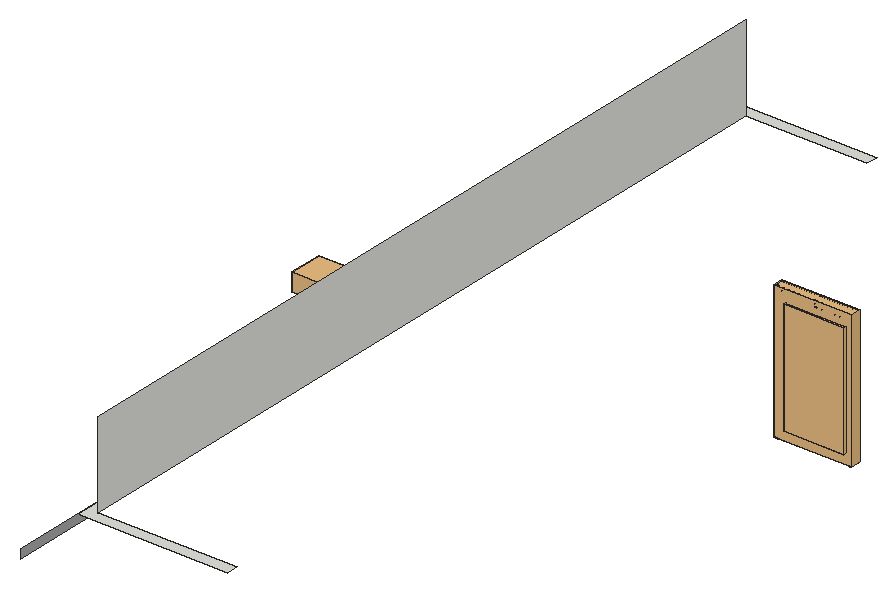
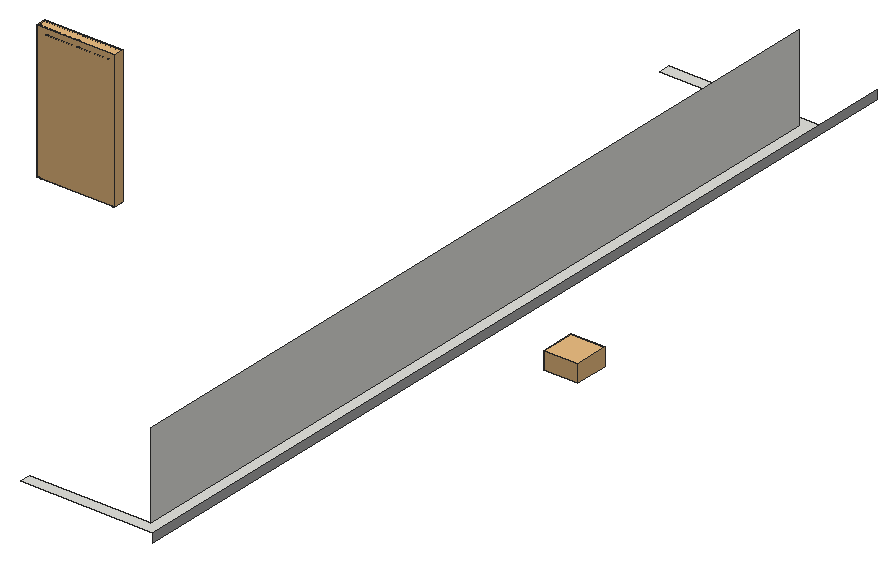
# SketchUp Ruby script. Lengths in inches.
U = 1.inch
M = Sketchup.active_model
def pt(a) = Geom::Point3d.new(a.map { |v| v * U })
def face(e, loops, mat)
  f = e.add_face(loops[0].map { |a| pt(a) })
  loops[1..].each { |l| e.add_face(l.map { |a| pt(a) }).erase! }
  f.material = f.back_material = mat if mat
  f
end
# faces: each face lists its corners as indices into pts; further lists are holes
def faces(e, pts, list, mat = nil) = list.each { |f| face(e, (f[0].is_a?(Array) ? f : [f]).map { |l| l.map { |i| pts[i] } }, mat) }
# xy, xz, yz: faces in a plane at the given z, y or x. An outline is a flat list of corners, or four numbers for a rectangle; further outlines are holes
def ring(l) = l.size == 4 ? [[l[0], l[1]], [l[2], l[1]], [l[2], l[3]], [l[0], l[3]]] : l.each_slice(2).to_a
def flat(e, list, mat, &to3) = list.each { |f| face(e, (f[0].is_a?(Array) ? f : [f]).map { |l| ring(l).map { |u, v| to3.(u, v) } }, mat) }
def xy(e, z, list, mat = nil) = flat(e, list, mat) { |x, y| [x, y, z] }
def xz(e, y, list, mat = nil) = flat(e, list, mat) { |x, z| [x, y, z] }
def yz(e, x, list, mat = nil) = flat(e, list, mat) { |y, z| [x, y, z] }
def lines(e, pts, list) = list.each { |a, b| e.add_line(pt(pts[a]), pt(pts[b])) }
# prism: a flat outline (further loops are holes) pulled along v
def prism(e, loops, v, mat = nil)
  f = face(e, loops, mat); d = Geom::Vector3d.new(v.map { |x| x * U })
  f.pushpull(f.normal.samedirection?(d) ? d.length : -d.length)
end
def box(e, o, s, mat = nil) = prism(e, [[o, [o[0] + s[0], o[1], o[2]], [o[0] + s[0], o[1] + s[1], o[2]], [o[0], o[1] + s[1], o[2]]]], [0, 0, s[2]], mat)
def at(x, y, z, deg = 0) = Geom::Transformation.translation(pt([x, y, z])) * Geom::Transformation.rotation(ORIGIN, Z_AXIS, deg.degrees)
def axes(o, x, y, z) = Geom::Transformation.new([*x, 0, *y, 0, *z, 0, *pt(o).to_a, 1])
def part(name) = M.definitions.add(name)
# library, detail: a bought-in or finely detailed component or shape, given as its bounding box
def library(name, o, s) = part(name).tap { |d| box(d.entities, o, s) }
def detail(e, o, s) = box(e.add_group.entities, o, s)
def put(e, d, t, mat = nil) = e.add_instance(d, t).tap { |i| i.material = mat if mat }
def group(e, t, mat = nil) = e.add_group.tap { |g| g.transformation = t; g.material = mat if mat }.entities
root = M.entities
M.materials.add("Material \#0").color = [86, 53, 35]
M.materials.add("Material \#1").color = [140, 140, 140]
M.materials.add("[0132_LightGray]").color = [169, 169, 169]
c1 = library("Dome Light",[-12,-12,0],[24,24,12])
c2 = part("3DGeom~18_Defintion")
xz(c2.entities,-241.71,[[-976.3,0,23.7,0,23.7,7.58],[-976.3,0,23.7,7.58,-976.3,7.58]],"Material \#0")
xz(c2.entities,241.71,[[-976.3,0,-976.3,7.58,23.7,7.58],[-976.3,0,23.7,7.58,23.7,0]],"Material \#0")
yz(c2.entities,23.7,[[-241.71,0,0,0,-241.71,7.58],[0,0,0,7.58,-241.71,7.58],[0,0,241.71,0,241.71,7.58],[0,0,241.71,7.58,0,7.58]],"Material \#0")
c3 = part("3DGeom~20_Defintion")
xy(c3.entities,0,[[-976.3,-241.71,-976.3,-223.46,23.7,-241.71],[23.7,-241.71,-976.3,-223.46,5.45,-223.46],[23.7,-241.71,5.45,-223.46,5.45,0],[23.7,-241.71,5.45,0,23.7,0],[-976.3,-223.46,-976.3,-211.85,5.45,-223.46],
  [5.45,-223.46,-976.3,-211.85,-6.16,-211.85],[5.45,-223.46,-6.16,-211.85,-6.16,0],[5.45,-223.46,-6.16,0,5.45,0],[-6.16,0,-6.16,211.85,5.45,223.46],[-6.16,0,5.45,223.46,5.45,0],
  [5.45,0,23.7,241.71,23.7,0],[5.45,0,5.45,223.46,23.7,241.71],[-976.3,211.85,-976.3,223.46,5.45,223.46],[-976.3,211.85,5.45,223.46,-6.16,211.85],[-976.3,223.46,-976.3,241.71,23.7,241.71],
  [-976.3,223.46,23.7,241.71,5.45,223.46]],"Material \#0")
c4 = part("3DGeom~22_Defintion")
xz(c4.entities,-210.625,[[-1016.13,2.47,-1016.13,9.96,-16.28,2.47],[-16.28,2.47,-1016.13,9.96,-16.28,9.96],[-1016.13,9.96,-1016.13,51.7,-16.28,51.7],[-1016.13,9.96,-16.28,51.7,-16.28,9.96],[-1016.13,51.7,-1016.13,72.71,-16.28,51.7]],"Material \#0")
xz(c4.entities,210.625,[[-1016.13,2.47,-16.28,2.47,-1016.13,9.96],[-16.28,2.47,-16.28,9.96,-1016.13,9.96],[-1016.13,9.96,-16.28,51.7,-1016.13,51.7],[-1016.13,9.96,-16.28,9.96,-16.28,51.7],[-1016.13,51.7,-16.28,51.7,-1016.13,72.71]],"Material \#0")
yz(c4.entities,-16.28,[[-210.625,2.47,-210.625,9.96,0,9.96],[-210.625,2.47,0,9.96,0,2.47],[0,2.47,0,9.96,210.625,2.47],[210.625,2.47,0,9.96,210.625,9.96],[-210.625,9.96,-210.625,51.7,0,51.7],
  [-210.625,9.96,0,51.7,0,9.96],[0,9.96,0,51.7,210.625,9.96],[210.625,9.96,0,51.7,210.625,51.7],[-210.625,51.7,0,72.71,0,51.7],[0,51.7,0,72.71,210.625,51.7]],"Material \#0")
p = [[-1016.13,-210.625,72.71],[-16.13,-210.77,73.09],[-16.28,-210.625,51.7],[-16.28,-210.625,51.7],[-16.13,-210.77,73.09],[-16.28,0,72.71],
  [-16.13,210.77,73.09],[-16.28,210.625,51.7],[-16.28,210.625,51.7],[-16.13,210.77,73.09],[-1016.13,210.625,72.71]]
faces(c4.entities,p,[[0,1,2],[3,4,5],[5,6,7],[8,9,10]],"Material \#0")
c5 = part("3DGeom~21_Defintion")
xy(c5.entities,73.08,[[-976.3,-241.71,23.7,-241.71,-976.3,-223.46],[23.7,-241.71,5.45,-223.46,-976.3,-223.46],[23.7,-241.71,23.7,0,5.45,-223.46],[5.45,-223.46,23.7,0,5.45,0],[23.7,0,23.7,241.71,5.45,223.46],
  [5.45,0,23.7,0,5.45,223.46],[-976.3,223.46,23.7,241.71,-976.3,241.71],[-976.3,223.46,5.45,223.46,23.7,241.71]],"Material \#0")
c6 = part("3DGeom~19_Defintion")
xy(c6.entities,0,[[-6.28,-215.79,-994.45,-208.55,-13.52,-208.55],[-994.45,-215.79,-994.45,-208.55,-6.28,-215.79],[-6.28,-215.79,-13.52,-208.55,-13.52,0],[-6.28,-215.79,-13.52,0,-6.28,0],[-13.52,0,-13.52,208.55,-6.28,215.79],
  [-13.52,0,-6.28,215.79,-6.28,0],[-994.45,208.55,-6.28,215.79,-13.52,208.55],[-994.45,208.55,-994.45,215.79,-6.28,215.79]],"Material \#0")
p = [[-13.52,-208.55,0],[-994.45,-208.55,0],[-994.45,-207.81,0.07],[-14.25,-207.81,0.07],[-13.52,-208.55,0],[-14.25,-207.81,0.07],
  [-14.25,0,0.07],[-13.52,0,0],[-13.52,208.55,0],[-14.25,207.81,0.07],[-13.52,208.55,0],[-14.25,207.81,0.07],
  [-994.45,207.81,0.07],[-994.45,208.55,0],[-994.45,-207.21,0.27],[-994.45,-207.21,0.27],[-14.86,-207.21,0.27],[-14.86,-207.21,0.27],
  [-14.86,0,0.27],[-14.86,0,0.27],[-14.86,0,0.27],[-14.86,0,0.27],[-14.86,207.21,0.27],[-14.86,207.21,0.27],
  [-994.45,207.21,0.27],[-994.45,207.21,0.27],[-14.86,-207.21,0.27],[-994.45,-207.21,0.27],[-994.45,-206.74,0.6],[-15.33,-206.74,0.6],
  [-14.86,-207.21,0.27],[-15.33,-206.74,0.6],[-15.33,0,0.6],[-14.86,0,0.27],[-14.86,207.21,0.27],[-15.33,206.74,0.6],
  [-14.86,207.21,0.27],[-15.33,206.74,0.6],[-994.45,206.74,0.6],[-994.45,207.21,0.27],[-994.45,-206.4,1.07],[-15.66,-206.4,1.07],
  [-15.66,-206.4,1.07],[-15.66,0,1.07],[-15.66,206.4,1.07],[-15.66,206.4,1.07],[-994.45,206.4,1.07],[-994.45,-206.2,1.68],
  [-15.86,-206.2,1.68],[-15.86,-206.2,1.68],[-15.86,0,1.68],[-15.86,206.2,1.68],[-15.86,206.2,1.68],[-994.45,206.2,1.68],
  [-994.45,-206.13,2.41],[-15.93,-206.13,2.41],[-15.93,-206.13,2.41],[-15.93,0,2.41],[-15.93,206.13,2.41],[-15.93,206.13,2.41],
  [-994.45,206.13,2.41],[-994.45,-206.13,71.16],[-994.45,-206.22,71.59],[-15.79,-206.28,71.53],[-15.79,-206.28,71.53],[-15.84,0,71.59],
  [-15.93,0,71.16],[-15.79,206.28,71.53],[-15.79,206.28,71.53],[-994.45,206.22,71.59],[-994.45,206.13,71.16],[-15.79,-206.28,71.53],
  [-994.45,-206.48,71.84],[-994.45,-206.9,71.93],[-15.16,-206.9,71.93],[-15.79,-206.28,71.53],[-15.79,-206.28,71.53],[-15.16,-206.9,71.93],
  [-15.16,0,71.93],[-994.45,-206.48,71.84],[-15.59,0,71.84],[-15.79,-206.28,71.53],[-15.59,0,71.84],[-15.79,206.28,71.53],
  [-15.16,206.9,71.93],[-15.59,0,71.84],[-15.79,206.28,71.53],[-994.45,206.48,71.84],[-15.79,206.28,71.53],[-15.16,206.9,71.93],
  [-994.45,206.9,71.93],[-994.45,206.48,71.84],[-15.79,206.28,71.53],[-994.45,-227.27,72.01],[5.41,-227.47,72.33],[4.78,-226.84,71.93],
  [4.78,-226.84,71.93],[5.41,-227.47,72.33],[5.21,0,72.01],[-994.45,-226.84,71.93],[-994.45,-227.27,72.01],[5.21,0,72.01],
  [4.78,0,71.93],[4.78,226.84,71.93],[5.21,0,72.01],[5.21,0,72.01],[5.41,227.47,72.33],[4.78,226.84,71.93],
  [5.41,227.47,72.33],[-994.45,227.27,72.01],[-994.45,227.27,72.01],[-994.45,226.84,71.93],[-994.45,-227.27,72.01],[-994.45,-227.53,72.27],
  [5.41,-227.47,72.33],[5.41,-227.47,72.33],[5.47,0,72.27],[5.21,0,72.01],[5.41,227.47,72.33],[5.41,227.47,72.33],
  [-994.45,227.53,72.27],[-994.45,227.27,72.01],[-994.45,-227.61,72.7],[-994.45,-227.61,74.4375],[-994.45,-227.61,74.4375],[5.55,-227.61,74.4375],
  [5.55,-227.61,74.4375],[5.55,0,74.4375],[5.55,0,72.7],[5.55,227.61,74.4375],[5.55,227.61,74.4375],[-994.45,227.61,74.4375],
  [-994.45,227.61,74.4375],[-994.45,227.61,72.7]]
faces(c6.entities,p,[[0,1,2],[2,3,0],[4,5,6],[6,7,4],[8,7,6],[6,9,8],[10,11,12],[12,13,10],
  [3,2,14],[15,16,3],[5,17,18],[19,6,5],[9,6,20],[21,22,9],[11,23,24],[25,12,11],
  [26,27,28],[28,29,26],[30,31,32],[32,33,30],[34,33,32],[32,35,34],[36,37,38],[38,39,36],
  [29,28,40],[40,41,29],[31,42,43],[43,32,31],[35,32,43],[43,44,35],[37,45,46],[46,38,37],
  [41,40,47],[47,48,41],[42,49,50],[50,43,42],[44,43,50],[50,51,44],[45,52,53],[53,46,45],
  [48,47,54],[54,55,48],[49,56,57],[57,50,49],[51,50,57],[57,58,51],[52,59,60],[60,53,52],
  [61,62,63],[64,65,66],[66,65,67],[68,69,70],[71,72,73],[73,74,75],[76,77,78],[62,79,63],
  [78,80,76],[81,82,65],[83,80,78],[78,84,83],[65,85,86],[68,87,69],[88,89,90],[90,91,92],
  [93,94,95],[96,97,98],[95,99,100],[101,102,96],[103,102,104],[105,106,103],[107,108,109],[110,111,107],
  [112,113,114],[115,116,117],[117,116,118],[119,120,121],[114,122,123],[124,125,114],[113,122,114],[115,126,127],
  [127,128,115],[115,128,116],[118,128,127],[127,129,118],[116,128,118],[119,130,131],[132,133,119],[119,133,120]],"Material \#0")
c7 = part("3DGeom~15_Defintion")
xy(c7.entities,0,[[-961.58,-251.9,-958.5,-248.8125,-961.58,-237.8],[-961.58,-251.9,28.8,-248.8125,-958.5,-248.8125],[-961.58,-251.9,36.25,-251.9,28.8,-248.8125],[36.25,-251.9,19.98,-239.99,28.8,-248.8125],[36.25,-251.9,22.16,-237.8,19.98,-239.99],
  [-958.5,-248.8125,-958.5,-237.8,-961.58,-237.8],[19.98,-239.99,22.16,-237.8,3.36,-223.37],[-958.5,-237.8,-958.5,-223.37,-961.58,-220.28],[-961.58,-237.8,-958.5,-237.8,-961.58,-220.28],[22.16,-237.8,4.64,-220.28,3.36,-223.37],
  [-958.5,-223.37,4.64,-220.28,-961.58,-220.28],[-958.5,-223.37,3.36,-223.37,4.64,-220.28],[5.29,-219.63,8.375,-218.35,5.29,0],[8.375,-218.35,8.375,0,5.29,0],[5.29,0,8.375,0,5.29,219.63],
  [8.375,0,8.375,218.35,5.29,219.63],[8.375,218.35,22.8125,237.15,5.29,219.63],[-961.58,220.28,-958.5,223.37,-961.58,237.8],[-961.58,220.28,3.36,223.37,-958.5,223.37],[-961.58,220.28,4.64,220.28,3.36,223.37],
  [4.64,220.28,19.98,239.99,3.36,223.37],[4.64,220.28,22.16,237.8,19.98,239.99],[-958.5,223.37,-958.5,237.8,-961.58,237.8],[-958.5,237.8,-958.5,248.8125,-961.58,251.9],[-961.58,237.8,-958.5,237.8,-961.58,251.9],
  [22.16,237.8,28.8,248.8125,19.98,239.99],[22.16,237.8,36.25,251.9,28.8,248.8125],[-958.5,248.8125,36.25,251.9,-961.58,251.9],[-958.5,248.8125,28.8,248.8125,36.25,251.9]],"Material \#0")
xy(c7.entities,7.48,[[-962.79,-238.36,23.37,-238.36,-962.79,-219.67],[23.37,-238.36,4.67,-219.67,-962.79,-219.67],[23.37,-238.36,23.37,0,4.67,-219.67],[4.67,-219.67,23.37,0,4.67,0],[23.37,0,23.37,238.36,4.67,219.67],
  [4.67,0,23.37,0,4.67,219.67],[-962.79,219.67,23.37,238.36,-962.79,238.36],[-962.79,219.67,4.67,219.67,23.37,238.36]],"Material \#0")
xy(c7.entities,63.5625,[[-962.79,-238.36,-962.79,-219.67,4.67,-219.67],[-962.79,-238.36,4.67,-219.67,23.37,-238.36],[23.37,-238.36,4.67,-219.67,23.37,0],[4.67,-219.67,4.67,0,23.37,0],[23.37,0,4.67,219.67,23.37,238.36],
  [4.67,0,4.67,219.67,23.37,0],[-962.79,219.67,-962.79,238.36,4.67,219.67],[4.67,219.67,-962.79,238.36,23.37,238.36]],"Material \#0")
xy(c7.entities,69.64,[[-962.79,-219.62,4.63,-219.62,-962.79,-200.32],[4.63,-219.62,-14.68,-200.32,-962.79,-200.32],[4.63,-219.62,4.63,0,-14.68,-200.32],[-14.68,-200.32,4.63,0,-14.68,0],[-14.68,0,4.63,0,-14.68,200.32],
  [4.63,0,4.63,219.62,-14.68,200.32],[-962.79,200.32,-14.68,200.32,4.63,219.62],[-962.79,200.32,4.63,219.62,-962.79,219.62]],"Material \#0")
xy(c7.entities,71.04,[[-961.58,-251.9,-958.5,-248.8125,28.8,-248.8125],[-961.58,-251.9,-961.58,-237.8,-958.5,-248.8125],[-961.58,-251.9,28.8,-248.8125,36.25,-251.9],[36.25,-251.9,19.98,-239.99,22.16,-237.8],[36.25,-251.9,28.8,-248.8125,19.98,-239.99],
  [-958.5,-248.8125,-961.58,-237.8,-958.5,-237.8],[19.98,-239.99,3.36,-223.37,22.16,-237.8],[-958.5,-237.8,-961.58,-220.28,-958.5,-223.37],[-961.58,-237.8,-961.58,-220.28,-958.5,-237.8],[22.16,-237.8,3.36,-223.37,4.64,-220.28],
  [-958.5,-223.37,-961.58,-220.28,4.64,-220.28],[-958.5,-223.37,4.64,-220.28,3.36,-223.37],[5.29,-219.63,5.29,0,8.375,-218.35],[8.375,-218.35,5.29,0,8.375,0],[5.29,0,5.29,219.63,8.375,0],
  [8.375,0,5.29,219.63,8.375,218.35],[8.375,218.35,5.29,219.63,22.8125,237.15],[-961.58,220.28,-958.5,223.37,3.36,223.37],[-961.58,220.28,-961.58,237.8,-958.5,223.37],[-961.58,220.28,3.36,223.37,4.64,220.28],
  [4.64,220.28,3.36,223.37,19.98,239.99],[4.64,220.28,19.98,239.99,22.16,237.8],[-958.5,223.37,-961.58,237.8,-958.5,237.8],[-958.5,237.8,-961.58,251.9,-958.5,248.8125],[-961.58,237.8,-961.58,251.9,-958.5,237.8],
  [22.16,237.8,19.98,239.99,28.8,248.8125],[22.16,237.8,28.8,248.8125,36.25,251.9],[-958.5,248.8125,-961.58,251.9,36.25,251.9],[-958.5,248.8125,36.25,251.9,28.8,248.8125]],"Material \#0")
xz(c7.entities,-238.36,[[-962.79,63.5625,23.37,63.5625,23.37,72.07],[-962.79,63.5625,23.37,72.07,-962.79,72.07]],"Material \#0")
xz(c7.entities,-219.67,[[-962.79,7.48,4.67,7.48,-962.79,63.5625],[4.67,7.48,4.67,63.5625,-962.79,63.5625]],"Material \#0")
xz(c7.entities,219.67,[[-962.79,7.48,-962.79,63.5625,4.67,7.48],[4.67,7.48,-962.79,63.5625,4.67,63.5625]],"Material \#0")
xz(c7.entities,238.36,[[-962.79,63.5625,-962.79,72.07,23.37,72.07],[-962.79,63.5625,23.37,72.07,23.37,63.5625]],"Material \#0")
yz(c7.entities,4.67,[[-219.67,7.48,0,7.48,-219.67,63.5625],[0,7.48,0,63.5625,-219.67,63.5625],[0,7.48,219.67,63.5625,0,63.5625],[0,7.48,219.67,7.48,219.67,63.5625]],"Material \#0")
yz(c7.entities,23.37,[[-238.36,63.5625,0,63.5625,-238.36,72.07],[0,63.5625,0,72.07,-238.36,72.07],[0,63.5625,238.36,63.5625,238.36,72.07],[0,63.5625,238.36,72.07,0,72.07]],"Material \#0")
p = [[36.9,-251.24,0],[37.21,0,-0.16],[34.125,0,-0.14],[36.9,251.24,0],[33.83,243.81,0.02],[33.83,-243.8,0.02],
  [22.8125,-237.15,0],[24.99,-234.97,-0.01],[5.375,-220.37,0],[23.37,-238.36,7.48],[4.67,-219.67,7.48],[4.67,-219.67,7.48],
  [23.37,-238.36,7.48],[23.37,-238.36,0],[4.67,-219.67,7.48],[23.37,-238.36,0],[5.375,-220.37,0],[5.375,-220.37,0],
  [23.37,-238.36,0],[5.29,-219.63,0],[8.375,-218.35,0],[-15.36,-199.64,1.62],[4.67,-219.67,7.48],[5.375,-220.37,0],
  [-13.8,-201.19,0.06],[5.375,-220.37,0],[5.375,-220.37,0],[-14.84,-200.15,0.58],[5.375,-220.37,0],[-13.8,-201.19,0.06],
  [-6.08,-208.92,0],[5.375,-220.37,0],[-13.8,-201.19,0.06],[-6.08,-208.92,0],[-13.8,-201.19,0.06],[5.375,-220.37,0],
  [-6.08,-208.92,0],[-13.8,-201.19,0.06],[-13.09,-201.91,0],[-6.08,-208.92,0],[-13.09,-201.91,0],[-13.8,-201.19,0.06],
  [-15.36,199.64,1.62],[4.67,219.67,7.48],[5.375,220.37,0],[-13.8,201.19,0.06],[5.375,220.37,0],[5.375,220.37,0],
  [4.67,219.67,7.48],[-14.84,200.15,0.58],[5.375,220.37,0],[-13.8,201.19,0.06],[-6.08,208.92,0],[-13.09,201.91,0],
  [-13.8,201.19,0.06],[-6.08,208.92,0],[-13.8,201.19,0.06],[5.375,220.37,0],[-6.08,208.92,0],[5.375,220.37,0],
  [-13.8,201.19,0.06],[-6.08,208.92,0],[-13.8,201.19,0.06],[-13.09,201.91,0],[8.375,218.35,0],[24.99,234.97,-0.01],
  [22.8125,237.15,0],[23.37,238.36,7.48],[23.37,238.36,0],[23.37,238.36,0],[5.375,220.37,0],[5.375,220.37,0],
  [23.37,238.36,7.48],[4.67,219.67,7.48],[5.375,220.37,0],[23.37,238.36,0],[23.37,238.36,7.48],[-13.8,-201.19,0.06],
  [-14.84,-200.15,0.58],[-14.38,-200.61,0.26],[-13.8,-201.19,0.06],[-13.8,-201.19,0.06],[-14.38,-200.61,0.26],[-13.8,201.19,0.06],
  [-14.84,200.15,0.58],[-13.8,201.19,0.06],[-14.38,200.61,0.26],[-14.38,200.61,0.26],[-13.8,201.19,0.06],[4.63,-219.62,69.64],
  [4.63,-219.62,69.64],[-15.42,-199.57,9.43],[-15.36,-199.64,1.62],[-15.16,-199.83,1.04],[-15.16,-199.83,1.04],[-15.16,199.83,1.04],
  [-15.36,199.64,1.62],[-15.16,199.83,1.04],[-15.42,199.57,9.43],[4.63,219.62,69.64],[4.67,219.67,7.48],[4.63,219.62,69.64],
  [4.63,-219.62,69.64],[4.67,-219.67,63.5625],[4.67,-219.67,63.5625],[4.67,-219.67,7.48],[-15.28,-199.71,69.25],[4.63,-219.62,69.64],
  [-15.42,-199.57,9.43],[-15.28,-199.71,69.25],[-15.42,-199.57,2.34],[-15.42,-199.57,2.34],[-15.42,199.57,2.34],[-15.42,199.57,9.43],
  [-15.28,199.71,69.25],[-15.28,199.71,69.25],[4.63,219.62,69.64],[4.63,219.62,69.64],[4.67,219.67,63.5625],[4.67,219.67,63.5625],
  [-15.42,199.57,2.34],[4.67,-219.67,63.5625],[4.63,-219.62,69.64],[4.67,219.67,7.48],[4.67,219.67,63.5625],[4.63,219.62,69.64],
  [4.63,-219.62,69.64],[-15.28,-199.71,69.25],[-15.28,-199.71,69.25],[-15.42,-199.57,48.99],[-15.42,-199.57,48.99],[-15.28,-199.71,69.25],
  [-15.42,199.57,48.99],[-15.28,199.71,69.25],[-15.28,199.71,69.25],[-15.42,199.57,48.99],[4.63,219.62,69.64],[4.63,-219.62,69.64],
  [23.37,-238.36,72.07],[4.67,-219.67,63.5625],[4.67,-219.67,63.5625],[23.37,-238.36,63.5625],[23.37,-238.36,72.07],[4.67,-219.67,63.5625],
  [5.24,-220.23,70.03],[23.37,-238.36,72.07],[23.37,-238.36,63.5625],[4.67,-219.67,63.5625],[4.67,-219.67,63.5625],[4.63,-219.62,69.64],
  [4.63,219.62,69.64],[23.37,238.36,72.07],[4.67,219.67,63.5625],[4.67,219.67,63.5625],[5.24,220.23,70.03],[4.63,219.62,69.64],
  [23.37,238.36,63.5625],[4.67,219.67,63.5625],[4.67,219.67,63.5625],[23.37,238.36,63.5625],[23.37,238.36,72.07],[4.67,219.67,63.5625],
  [23.37,238.36,72.07],[4.63,-219.62,69.64],[-14.68,-200.32,69.64],[-15.28,-199.71,69.25],[-15.28,-199.71,69.25],[-14.68,-200.32,69.64],
  [4.63,-219.62,69.64],[-15.28,199.71,69.25],[-14.68,200.32,69.64],[4.63,219.62,69.64],[4.63,219.62,69.64],[-14.68,200.32,69.64],
  [4.63,-219.62,69.64],[5.24,-220.23,70.03],[23.37,-238.36,72.07],[4.63,219.62,69.64],[5.24,220.23,70.03],[5.375,-220.37,72.07],
  [5.375,-220.37,72.07],[23.37,-238.36,72.07],[5.375,220.37,72.07],[23.37,238.36,72.07],[5.375,220.37,72.07],[33.83,-243.8,71.03],
  [36.9,-251.24,71.04],[22.8125,-237.15,71.04],[34.125,0,71.19],[37.21,0,71.2],[24.99,-234.97,71.05],[5.29,-219.63,71.04],
  [8.375,-218.35,71.04],[33.83,243.81,71.03],[36.9,251.24,71.04],[22.8125,237.15,71.04],[24.99,234.97,71.05],[8.375,218.35,71.04]]
faces(c7.entities,p,[[0,1,2],[1,3,4],[4,2,1],[2,5,0],[6,0,5],[5,7,6],[8,9,10],[11,12,13],
  [14,15,16],[17,18,9],[19,6,7],[7,20,19],[21,22,23],[24,21,25],[26,10,27],[28,27,29],
  [30,31,32],[33,34,35],[36,37,38],[39,40,41],[42,43,44],[45,42,46],[47,48,49],[50,49,51],
  [52,53,54],[55,56,57],[58,59,60],[61,62,63],[64,65,66],[43,67,68],[43,69,70],[71,72,73],
  [74,75,76],[3,66,65],[65,4,3],[77,78,21],[27,79,80],[81,82,78],[83,84,42],[85,86,84],
  [49,87,88],[10,89,27],[90,91,27],[92,93,27],[91,92,27],[78,94,21],[84,95,42],[96,97,49],
  [98,96,49],[99,98,49],[100,101,49],[21,102,103],[21,104,105],[21,106,107],[21,108,109],[91,110,92],
  [21,111,108],[42,112,113],[42,113,114],[42,115,116],[42,117,118],[42,119,43],[98,120,96],[10,121,122],
  [123,124,125],[126,127,91],[128,129,91],[108,130,131],[113,132,133],[134,135,98],[136,134,98],[137,138,139],
  [140,141,142],[143,142,144],[145,146,147],[148,144,149],[150,151,152],[153,154,155],[151,156,157],[158,159,160],
  [161,162,154],[163,164,165],[166,167,168],[169,170,171],[172,173,134],[174,175,176],[177,178,151],[142,179,144],
  [175,180,181],[178,182,151],[183,184,154],[185,186,187],[186,185,188],[188,189,186],[187,190,185],[190,187,191],
  [191,192,190],[189,188,193],[193,194,189],[195,196,197],[196,195,194],[194,193,196]],"Material \#0")
c8 = library("3DGeom~16_Defintion",[-962.62,-252.34,-11.22],[1000,504.68,93.46])
c9 = part("3DGeom~17_Defintion")
yz(c9.entities,-1908.8,[[-436.03,-21.87,-436.73,-21.5,-435.91,-21.83],[436.03,-21.87,435.91,-21.83,436.73,-21.5],[-435.91,-21.83,-436.73,-21.5,-436.15,-21.125],[-435.91,-21.83,-436.15,-21.125,-435.87,-21.72],[435.91,-21.83,435.87,-21.72,436.15,-21.125],
  [435.91,-21.83,436.15,-21.125,436.73,-21.5],[-436.73,-21.5,-484.73,-21.37,-436.15,-1.11],[-471.46,-21.5,-484.73,-21.37,-436.73,-21.5],[-477.2,-21.5,-484.73,-21.37,-471.46,-21.5],[-481.82,-21.5,-484.73,-21.37,-477.2,-21.5],
  [-436.73,-21.5,-436.15,-1.11,-436.15,-21.125],[436.73,-21.5,436.15,-21.125,471.46,-21.5],[471.46,-21.5,436.15,-21.125,477.2,-21.5],[477.2,-21.5,436.15,-21.125,499.98,-0.85],[477.2,-21.5,499.98,-0.85,481.82,-21.5],
  [481.82,-21.5,487.35,-21,484.73,-21.37],[481.82,-21.5,491.8,-19.52,487.35,-21],[481.82,-21.5,497.64,-13.67,491.8,-19.52],[481.82,-21.5,499.98,-0.85,497.64,-13.67],[-484.73,-21.37,-498.5,-11.58,-499.84,-0.37],
  [-484.73,-21.37,-499.84,-0.37,-499.4,-0.5],[-484.73,-21.37,-499.4,-0.5,-436.15,-1.11],[-484.73,-21.37,-493.63,-18.42,-498.5,-11.58],[-484.73,-21.37,-489.71,-20.375,-493.63,-18.42],[-484.73,-21.37,-487.35,-21,-489.71,-20.375],
  [436.15,-21.125,436.15,-1.11,436.73,-0.74],[436.15,-21.125,436.73,-0.74,499.98,-0.85],[487.35,-21,491.8,-19.52,489.71,-20.375],[-489.71,-20.375,-491.8,-19.52,-493.63,-18.42],[491.8,-19.52,495.21,-17.08,493.63,-18.42],
  [491.8,-19.52,497.64,-13.67,495.21,-17.08],[-493.63,-18.42,-496.54,-15.5,-498.5,-11.58],[-493.63,-18.42,-495.21,-17.08,-496.54,-15.5],[495.21,-17.08,497.64,-13.67,496.54,-15.5],[-496.54,-15.5,-497.64,-13.67,-498.5,-11.58],
  [497.64,-13.67,499.125,-9.22,498.5,-11.58],[497.64,-13.67,499.625,-3.69,499.125,-9.22],[497.64,-13.67,499.98,-0.85,499.625,-3.69],[-498.5,-11.58,-499.625,-3.69,-499.84,-0.37],[-498.5,-11.58,-499.5,-6.6,-499.625,-3.69],
  [-498.5,-11.58,-499.125,-9.22,-499.5,-6.6],[499.125,-9.22,499.625,-3.69,499.5,-6.6],[-499.625,-3.69,-499.98,-0.85,-500,-0.52],[-499.625,-3.69,-500,-0.52,-499.84,-0.37],[-436.15,-1.11,-499.4,-0.5,-471.46,-0.74],
  [-436.15,-1.11,-471.46,-0.74,-436.73,-0.74],[-436.15,-1.11,-436.73,-0.74,-435.91,-0.41],[-436.15,-1.11,-435.91,-0.41,-435.87,-0.52],[436.15,-1.11,435.87,-0.52,435.91,-0.41],[436.15,-1.11,435.91,-0.41,436.73,-0.74],
  [499.98,-0.85,436.73,-0.74,471.46,-0.74],[499.98,-0.85,471.46,-0.74,499.4,-0.5],[499.98,-0.85,499.4,-0.5,499.96,-0.41],[499.98,-0.85,499.96,-0.41,500,-0.52],[-436.73,-0.74,-436.03,-0.37,-435.91,-0.41],
  [436.73,-0.74,435.91,-0.41,436.03,-0.37],[-500,-0.52,-499.96,-0.41,-499.84,-0.37],[499.4,-0.5,499.84,-0.37,499.96,-0.41],[-499.84,141.21,-499.96,141.25,-499.4,141.35],[-436.03,141.21,-436.73,141.59,-435.91,141.25],
  [436.03,141.21,435.91,141.25,436.73,141.59],[499.84,141.21,484.73,162.21,498.5,152.42],[499.84,141.21,499.4,141.35,484.73,162.21],[499.84,141.21,498.5,152.42,499.625,144.53],[499.84,141.21,499.625,144.53,500,141.37],
  [499.84,141.21,500,141.37,499.96,141.25],[-499.96,141.25,-500,141.37,-499.98,141.69],[-499.96,141.25,-499.98,141.69,-499.4,141.35],[-435.91,141.25,-436.73,141.59,-436.15,141.96],[-435.91,141.25,-436.15,141.96,-435.87,141.37],
  [435.91,141.25,435.87,141.37,436.15,141.96],[435.91,141.25,436.15,141.96,436.73,141.59],[-499.4,141.35,-499.98,141.69,-471.46,141.59],[499.4,141.35,436.15,141.96,484.73,162.21],[499.4,141.35,471.46,141.59,436.15,141.96],
  [500,141.37,499.625,144.53,499.98,141.69],[-436.73,141.59,-499.98,141.69,-436.15,161.97],[-471.46,141.59,-499.98,141.69,-436.73,141.59],[-436.73,141.59,-436.15,161.97,-436.15,141.96],[436.73,141.59,436.15,141.96,471.46,141.59],
  [-499.98,141.69,-477.2,162.34,-436.15,161.97],[-499.98,141.69,-481.82,162.34,-477.2,162.34],[-499.98,141.69,-497.64,154.51,-481.82,162.34],[-499.98,141.69,-499.625,144.53,-497.64,154.51],[436.15,141.96,436.15,161.97,436.73,162.34],
  [436.15,141.96,436.73,162.34,484.73,162.21],[-499.625,144.53,-499.125,150.07,-497.64,154.51],[-499.625,144.53,-499.5,147.44,-499.125,150.07],[499.625,144.53,498.5,152.42,499.5,147.44],[499.5,147.44,498.5,152.42,499.125,150.07],
  [-499.125,150.07,-498.5,152.42,-497.64,154.51],[498.5,152.42,484.73,162.21,493.63,159.26],[498.5,152.42,493.63,159.26,496.54,156.34],[498.5,152.42,496.54,156.34,497.64,154.51],[-497.64,154.51,-491.8,160.36,-481.82,162.34],
  [-497.64,154.51,-495.21,157.92,-491.8,160.36],[-497.64,154.51,-496.54,156.34,-495.21,157.92],[496.54,156.34,493.63,159.26,495.21,157.92],[-495.21,157.92,-493.63,159.26,-491.8,160.36],[493.63,159.26,484.73,162.21,489.71,161.22],
  [493.63,159.26,489.71,161.22,491.8,160.36],[-491.8,160.36,-487.35,161.84,-481.82,162.34],[-491.8,160.36,-489.71,161.22,-487.35,161.84],[489.71,161.22,484.73,162.21,487.35,161.84],[-487.35,161.84,-484.73,162.21,-481.82,162.34],
  [-436.15,161.97,-477.2,162.34,-471.46,162.34],[-436.15,161.97,-471.46,162.34,-436.73,162.34],[-436.15,161.97,-436.73,162.34,-435.91,162.68],[-436.15,161.97,-435.91,162.68,-435.87,162.56],[436.15,161.97,435.87,162.56,435.91,162.68],
  [436.15,161.97,435.91,162.68,436.73,162.34],[484.73,162.21,436.73,162.34,471.46,162.34],[484.73,162.21,471.46,162.34,477.2,162.34],[484.73,162.21,477.2,162.34,481.82,162.34],[-436.73,162.34,-436.03,162.72,-435.91,162.68],
  [436.73,162.34,435.91,162.68,436.03,162.72]],"Material \#0")
c10 = library("3DGeom~6_Defintion",[-5.59,-471.8,-48.03],[468.87,1000,73.72])
xy(root,0,[[1338.625,223.9375,1338.625,807.5,1431.3125,807.5,1431.3125,799.5,1346.625,799.5,1346.625,231.9375,1443.61,231.9375,1443.61,223.9375]])
yz(root,1338.625,[[173.9375,-6,807.5,0]],"[0132_LightGray]")
yz(root,1346.625,[[231.9375,0,799.5,60]])
put(root,c1,at(1280.26,511.33,-6))
put(root,c2,axes([1609.42,535.42,91.6875],[0,0,0.09391],[0.10549,0,0],[0,-0.07326,0]),"Material \#0")
put(root,c3,axes([1609.42,535.42,91.6875],[0,0,0.09391],[0.10549,0,0],[0,-0.07326,0]),"Material \#0")
put(root,c4,axes([1609.42,535.42,91.6875],[0,0,0.09023],[0.10136,0,0],[0,-0.07039,0]),"Material \#0")
put(root,c5,axes([1609.42,535.42,91.6875],[0,0,0.09391],[0.10549,0,0],[0,-0.07326,0]),"Material \#0")
put(root,c6,axes([1609.42,535.42,91.6875],[0,0,0.0922],[0.10357,0,0],[0,-0.07192,0]),"Material \#0")
put(root,c7,axes([1609.42,535.42,91.6875],[0,0,0.09523],[0.10697,0,0],[0,-0.07429,0]),"Material \#0")
put(root,c8,axes([1609.42,535.42,91.6875],[0,0,0.09525],[0.10699,0,0],[0,-0.0743,0]),"Material \#0")
put(root,c9,axes([1609.42,535.42,91.6875],[0,0,0.04803],[0.05396,0,0],[0,-0.03747,0]),"Material \#0")
put(root,c10,axes([1590.92,531.05,44.51],[0.08952,0,0],[0,0,0.07969],[0,0.06217,0]),"Material \#1")
